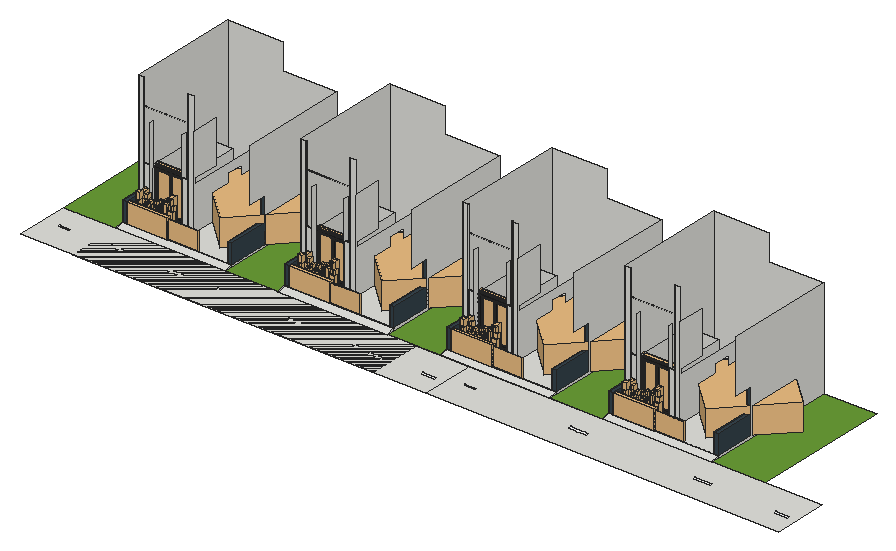
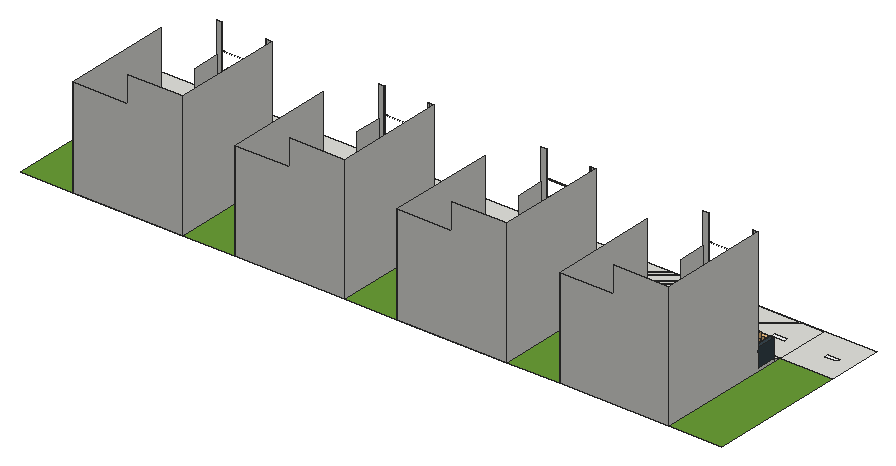
# SketchUp Ruby script. Lengths in inches.
U = 1.inch
M = Sketchup.active_model
def pt(a) = Geom::Point3d.new(a.map { |v| v * U })
def face(e, loops, mat)
  f = e.add_face(loops[0].map { |a| pt(a) })
  loops[1..].each { |l| e.add_face(l.map { |a| pt(a) }).erase! }
  f.material = f.back_material = mat if mat
  f
end
# faces: each face lists its corners as indices into pts; further lists are holes
def faces(e, pts, list, mat = nil) = list.each { |f| face(e, (f[0].is_a?(Array) ? f : [f]).map { |l| l.map { |i| pts[i] } }, mat) }
# xy, xz, yz: faces in a plane at the given z, y or x. An outline is a flat list of corners, or four numbers for a rectangle; further outlines are holes
def ring(l) = l.size == 4 ? [[l[0], l[1]], [l[2], l[1]], [l[2], l[3]], [l[0], l[3]]] : l.each_slice(2).to_a
def flat(e, list, mat, &to3) = list.each { |f| face(e, (f[0].is_a?(Array) ? f : [f]).map { |l| ring(l).map { |u, v| to3.(u, v) } }, mat) }
def xy(e, z, list, mat = nil) = flat(e, list, mat) { |x, y| [x, y, z] }
def xz(e, y, list, mat = nil) = flat(e, list, mat) { |x, z| [x, y, z] }
def yz(e, x, list, mat = nil) = flat(e, list, mat) { |y, z| [x, y, z] }
def lines(e, pts, list) = list.each { |a, b| e.add_line(pt(pts[a]), pt(pts[b])) }
# prism: a flat outline (further loops are holes) pulled along v
def prism(e, loops, v, mat = nil)
  f = face(e, loops, mat); d = Geom::Vector3d.new(v.map { |x| x * U })
  f.pushpull(f.normal.samedirection?(d) ? d.length : -d.length)
end
def box(e, o, s, mat = nil) = prism(e, [[o, [o[0] + s[0], o[1], o[2]], [o[0] + s[0], o[1] + s[1], o[2]], [o[0], o[1] + s[1], o[2]]]], [0, 0, s[2]], mat)
def at(x, y, z, deg = 0) = Geom::Transformation.translation(pt([x, y, z])) * Geom::Transformation.rotation(ORIGIN, Z_AXIS, deg.degrees)
def axes(o, x, y, z) = Geom::Transformation.new([*x, 0, *y, 0, *z, 0, *pt(o).to_a, 1])
def part(name) = M.definitions.add(name)
# library, detail: a bought-in or finely detailed component or shape, given as its bounding box
def library(name, o, s) = part(name).tap { |d| box(d.entities, o, s) }
def detail(e, o, s) = box(e.add_group.entities, o, s)
def put(e, d, t, mat = nil) = e.add_instance(d, t).tap { |i| i.material = mat if mat }
def group(e, t, mat = nil) = e.add_group.tap { |g| g.transformation = t; g.material = mat if mat }.entities
root = M.entities
M.materials.add("1480 AP K099 Starless Night-N").color = [54, 68, 77]
M.materials.add("BANANA_BIG_STVOL_1").color = [93, 83, 53]
M.materials.add("Color_000").color = [255, 255, 255]
M.materials.add("Material60").color = [234, 198, 157]
M.materials.add("POT_TEXTURE_1").color = [172, 172, 172]
M.materials.add("POT_TEXTURE_2").color = [160, 154, 144]
M.materials.add("[Color_009]").color = [33, 33, 33]
M.materials.add("[Color_A01]").color = [253, 112, 112]
M.materials["[Color_A01]"].alpha = 0
M.materials.add("[Grass Dark Green]").color = [106, 157, 55]
M.materials.add("soil1").color = [68, 55, 47]
M.materials.add("wood_1").color = [140, 119, 94]
c1 = part("Untitled")
xy(c1.entities,0,[[[158.81,26.5625,306.06,993.3125],[225.28,357.51,237.28,411.51],[239.71,931.55,251.46,972.3],[233.64,703.93,242.14,755.18],[222.04,66.5,231.29,100.5]]])
xy(c1.entities,0,[[222.04,66.5,231.29,100.5],[225.28,357.51,237.28,411.51],[233.64,703.93,242.14,755.18],[239.71,931.55,251.46,972.3]],"Color_000")
c2 = part("Group\#163")
xy(c2.entities,0,[[0,0,144,382]],"[Grass Dark Green]")
c3 = part("Group\#161")
prism(c3.entities,[[[0,22,6],[0,22,0],[0,0,0]]],[300,0,0])
c4 = library("RANGE ROVER",[-63.71,-35.21,42.76],[182.88,182.88,64.08])
c5 = part("Bilal architect uae abu dhabi ")
put(c5.entities,c4,axes([104.22,-10.75,-48.75],[0.98727,0.57,0],[-0.57,0.98727,0],[0,0,1.14]),"Material60")
c6 = part("Group\#33")
prism(c6.entities,[[[22.64,0,0],[0,0,0],[0,43.31,0],[22.64,43.31,0]],[[20.67,41.34,0],[1.97,41.34,0],[1.97,1.97,0],[20.67,1.97,0]]],[0,0,1.38])
c7 = part("Group\#34")
box(c7.entities,[0,0,0],[18.7,39.37,0.39])
c8 = part("2slidwin w fix bottom")
put(c8.entities,c6,axes([1.97,0,22.15],[1,0,0],[0,0,1.25],[0,-1,0]),"[Color_009]")
put(c8.entities,c7,axes([3.9375,-0.2,24.61],[1,0,0],[0,0,1.25],[0,-1,0]),"[Color_A01]")
g1 = group(c8.entities,at(0,-0.2,0),"[Color_009]")
prism(g1,[[[47.24,0,19.69],[0,0,19.69],[0,0,78.74],[47.24,0,78.74]],[[45.28,0,22.15],[45.28,0,76.28],[1.97,0,76.28],[1.97,0,22.15]]],[0,-3.15,0])
put(c8.entities,c6,axes([22.64,-1.38,22.15],[1,0,0],[0,0,1.25],[0,-1,0]),"[Color_009]")
put(c8.entities,c7,axes([24.61,-1.57,24.61],[1,0,0],[0,0,1.25],[0,-1,0]),"[Color_A01]")
c9 = library("door by lz",[5.91,-4.92,0],[35.43,6.61,78.74])
c10 = library("Modern Gate 1",[0,0,0],[118.11,1.97,78.74])
c11 = library("Window_Curtains2",[0,-81.89,0],[92,82.37,8.12])
c12 = library("Group\#7",[0,-1,0],[111.5625,10,53])
c13 = part("Group")
box(c13.entities,[0,0,0],[12,55.4375,53])
c14 = part("Group\#6")
box(c14.entities,[0,0,0],[12,112.0625,53])
c15 = library("Group\#137",[-640.625,-1318.37,287.11],[396.64,314.81,689.96])
c16 = library("Group\#132",[-513.94,-1201.2,195.17],[480.66,557.42,1160.08])
c17 = library("Group\#134",[-208.03,-1336.63,286.21],[381.72,484.79,1145.39])
c18 = library("Group\#140",[-619.83,-1636.3,288.9],[316.15,456.61,1171.28])
c19 = library("Group\#141",[-738.91,-1210.08,301],[426.4,388.88,1000.79])
c20 = library("Group\#143",[-208.33,-1511.76,297.04],[508.2,421.96,1258.76])
c21 = library("Group\#133",[-545.36,-1775.03,287.125],[412.21,432,920.68])
c22 = library("Group\#138",[-750.24,-1478.51,301.56],[423.84,451.05,998.69])
c23 = library("Group\#136",[-245.33,-1174.2,301.22],[356.02,306.31,608.34])
c24 = library("Group\#131",[-487.23,-1483.58,-4.71],[450.86,446.99,418.38])
c25 = library("Group\#145",[-445.7,-1606.55,154.18],[255.44,283.57,849.28])
c26 = library("Group\#146",[-390.1,-1177.12,195.59],[220.93,265.44,790.12])
c27 = library("Group\#148",[-480.32,-1333.42,295.8],[424.49,356.06,1482.77])
c28 = library("Group\#149",[-378.01,-1245.98,305.66],[422.15,474.55,1267.42])
c29 = library("Group\#135",[-163.65,-1622.09,292.29],[406.18,374.8,780.12])
c30 = library("Group\#144",[-384.8,-1640.99,300.61],[422.68,348.03,1297.96])
c31 = library("Group\#130",[-429.18,-1441.17,362.05],[345.84,348.28,45.35])
c32 = library("Group\#147",[-208.0625,-1498.77,286.27],[547.26,435.76,1075.6])
c33 = library("Group\#142",[-172.82,-1329.68,294.68],[502.85,397.72,955.79])
c34 = library("Group\#139",[-426.76,-1753.59,287.48],[479.67,412.35,1049.19])
c35 = part("Potted palm")
put(c35.entities,c15,at(750.24,1775.03,4.71))
put(c35.entities,c16,at(750.24,1775.03,4.71))
put(c35.entities,c17,at(750.24,1775.03,4.71))
put(c35.entities,c18,at(750.24,1775.03,4.71))
put(c35.entities,c19,at(750.24,1775.03,4.71))
put(c35.entities,c20,at(750.24,1775.03,4.71))
put(c35.entities,c21,at(750.24,1775.03,4.71))
put(c35.entities,c22,at(750.24,1775.03,4.71))
put(c35.entities,c23,at(750.24,1775.03,4.71))
put(c35.entities,c24,at(750.24,1775.03,4.71),"POT_TEXTURE_1")
put(c35.entities,c25,at(750.24,1775.03,4.71))
put(c35.entities,c26,at(750.24,1775.03,4.71))
put(c35.entities,c27,at(750.24,1775.03,4.71))
put(c35.entities,c28,at(750.24,1775.03,4.71))
put(c35.entities,c29,at(750.24,1775.03,4.71))
put(c35.entities,c30,at(750.24,1775.03,4.71))
put(c35.entities,c31,at(750.24,1775.03,4.71),"soil1")
put(c35.entities,c32,at(750.24,1775.03,4.71))
put(c35.entities,c33,at(750.24,1775.03,4.71))
put(c35.entities,c34,at(750.24,1775.03,4.71))
c36 = library("Group\#96",[-662.41,217.3,320.04],[397.32,658.3,1732.06])
c37 = library("Group\#98",[-299.2,181.55,262.58],[360.65,735.71,1258.34])
c38 = library("Group\#93",[-1038.76,656.55,345.34],[733.18,460.51,2065.7])
c39 = library("Group\#91",[-445.29,890.31,329.28],[284.3,304.08,2023.29])
c40 = library("Group\#94",[-733.48,439.625,202.64],[456.28,533.12,1536.78])
c41 = library("Group\#97",[-455.56,899.32,410.78],[341.21,610.33,1581.5])
c42 = library("Group\#90",[-516.34,626.77,-4.5625],[517.73,515.95,418.98])
c43 = library("Group\#95",[-249.24,914.85,310.18],[345.55,647.95,1307.93])
c44 = library("Group\#92",[-277.97,488.68,287.26],[362.84,405.94,1768.54])
c45 = library("Group\#89",[-468.76,669.89,380.1875],[424.36,427.47,41.99])
c46 = part("Potted broadleaf plant")
put(c46.entities,c36,at(1038.76,-181.55,4.5625))
put(c46.entities,c37,at(1038.76,-181.55,4.5625))
put(c46.entities,c38,at(1038.76,-181.55,4.5625))
put(c46.entities,c39,at(1038.76,-181.55,4.5625))
put(c46.entities,c40,at(1038.76,-181.55,4.5625))
put(c46.entities,c41,at(1038.76,-181.55,4.5625))
put(c46.entities,c42,at(1038.76,-181.55,4.5625),"POT_TEXTURE_1")
put(c46.entities,c43,at(1038.76,-181.55,4.5625))
put(c46.entities,c44,at(1038.76,-181.55,4.5625))
put(c46.entities,c45,at(1038.76,-181.55,4.5625),"soil1")
c47 = library("Group\#102",[-246.45,-349.05,558.47],[136.91,100.49,66.1])
c48 = library("Group\#105",[-264.68,-415.73,1484.11],[304.64,209.69,227.41])
c49 = library("Group\#112",[-357.04,-394.18,1447.05],[213.62,306.36,356.95])
c50 = library("Group\#100",[-447.02,-464.95,536.35],[343.73,346.24,39.39])
c51 = library("Group\#101",[-394.9,-448.99,911.74],[90.19,96.88,85.93])
c52 = library("Group\#111",[-424,-312.27,817.53],[158.81,108.06,136.45])
c53 = library("Group\#115",[-409.02,-515.05,915.53],[69.62,77.27,65.47])
c54 = library("Group\#119",[-548.25,-262.82,1459.54],[373.26,352.35,568])
c55 = library("Group\#129",[-492.14,-508.4,-4.15],[433.72,431.71,567.03])
c56 = library("Group\#122",[-293.78,-482.77,597.9],[158.75,112.78,159.87])
c57 = library("Group\#106",[-545.09,-386.51,922.3125],[300.25,219.65,227.33])
c58 = library("Group\#127",[-292.81,-667.38,1418.14],[215.17,356.07,188.87])
c59 = library("Group\#108",[-292.14,-288.9,1281.79],[169.55,204.34,203.36])
c60 = library("Group\#113",[-568.91,-444.37,1285.4],[307.6,179.39,277.93])
c61 = library("Group\#110",[-341.93,-403.49,744.8125],[64.83,96.32,132.15])
c62 = library("Group\#99",[-258.04,-282.68,604.05],[115.53,137.01,52.63])
c63 = library("Group\#107",[-304.79,-269.16,622.65],[82.06,111.89,102.57])
c64 = library("Group\#114",[-388.93,-514.39,838.93],[89.79,77.73,82.08])
c65 = library("Group\#116",[-295.03,-516.52,742.34],[68.71,141.75,78.67])
c66 = library("Group\#123",[-422.77,-235.4,843.61],[178.54,197.77,233.54])
c67 = library("Group\#117",[-498.98,-524.4,908.45],[120.83,107.95,112.98])
c68 = library("Group\#120",[-321.08,-139.66,1308.49],[285.55,393.29,221.53])
c69 = library("Group\#118",[-278.4,-571.99,1530.91],[311.57,345.77,423.62])
c70 = library("Group\#121",[-387.74,-136.11,1470.07],[230,321.58,230.27])
c71 = library("Group\#109",[-244.55,-305.59,1009.46],[103.13,76.81,77.34])
c72 = library("Group\#128",[-385.21,-446.52,494.02],[160.93,321.12,1142.36])
c73 = library("Group\#103",[-249.18,-250.59,980.93],[152.21,116.16,134.05])
c74 = library("Group\#104",[-438.92,-265.61,702.3],[171.52,146.16,133.5])
c75 = part("Potted broadleaf tree")
p = [[568.91,667.38,4.15],[569.91,667.38,4.15],[569.91,668.38,4.15]]
lines(c75.entities,p,[[0,1],[1,2],[2,0]])
put(c75.entities,c47,at(568.91,667.38,4.15))
put(c75.entities,c48,at(568.91,667.38,4.15))
put(c75.entities,c49,at(568.91,667.38,4.15))
put(c75.entities,c50,at(568.91,667.38,4.15),"soil1")
put(c75.entities,c51,at(568.91,667.38,4.15))
put(c75.entities,c52,at(568.91,667.38,4.15))
put(c75.entities,c53,at(568.91,667.38,4.15))
put(c75.entities,c54,at(568.91,667.38,4.15))
put(c75.entities,c55,at(568.91,667.38,4.15),"POT_TEXTURE_2")
put(c75.entities,c56,at(568.91,667.38,4.15))
put(c75.entities,c57,at(568.91,667.38,4.15))
put(c75.entities,c58,at(568.91,667.38,4.15))
put(c75.entities,c59,at(568.91,667.38,4.15))
put(c75.entities,c60,at(568.91,667.38,4.15))
put(c75.entities,c61,at(568.91,667.38,4.15))
put(c75.entities,c62,at(568.91,667.38,4.15))
put(c75.entities,c63,at(568.91,667.38,4.15))
put(c75.entities,c64,at(568.91,667.38,4.15))
put(c75.entities,c65,at(568.91,667.38,4.15))
put(c75.entities,c66,at(568.91,667.38,4.15))
put(c75.entities,c67,at(568.91,667.38,4.15))
put(c75.entities,c68,at(568.91,667.38,4.15))
put(c75.entities,c69,at(568.91,667.38,4.15))
put(c75.entities,c70,at(568.91,667.38,4.15))
put(c75.entities,c71,at(568.91,667.38,4.15))
put(c75.entities,c72,at(568.91,667.38,4.15),"wood_1")
put(c75.entities,c73,at(568.91,667.38,4.15))
put(c75.entities,c74,at(568.91,667.38,4.15))
c76 = library("Group\#150",[-480.3,-2300.47,677.45],[398.14,398.43,28.25])
c77 = library("Group\#151",[-336.38,-2175.79,614.41],[133.99,147.1,560.64])
c78 = library("Group\#152",[-311.45,-2362.85,663.67],[597.01,322.07,1007.38])
c79 = library("Group\#153",[-330.26,-2159.14,612.04],[116.66,119.22,673.97])
c80 = library("Group\#154",[-667.53,-2111.4375,1071.74],[420.02,555.28,968.03])
c81 = library("Group\#155",[-328.97,-2115.58,1156.29],[117.86,119.42,695.38])
c82 = library("Group\#156",[-943.22,-2312.1875,967.59],[670.63,402.45,1245.73])
c83 = library("Group\#158",[-343.93,-2076.42,1024.91],[285.05,475.82,708.21])
c84 = library("Group\#157",[-568.09,-2386.9,-3.76],[573.62,569.18,700.28])
c85 = library("Group\#159",[-550.09,-2664.39,1031.96],[371.42,533.86,798])
c86 = library("Group\#160",[-308.37,-2556.11,869.35],[483.58,483.6,1385.8])
c87 = part("Potted broadleaf plant \#1")
put(c87.entities,c76,at(943.22,2664.39,3.76),"soil1")
put(c87.entities,c77,at(943.22,2664.39,3.76),"BANANA_BIG_STVOL_1")
put(c87.entities,c78,at(943.22,2664.39,3.76))
put(c87.entities,c79,at(943.22,2664.39,3.76),"BANANA_BIG_STVOL_1")
put(c87.entities,c80,at(943.22,2664.39,3.76))
put(c87.entities,c81,at(943.22,2664.39,3.76))
put(c87.entities,c82,at(943.22,2664.39,3.76))
put(c87.entities,c83,at(943.22,2664.39,3.76))
put(c87.entities,c84,at(943.22,2664.39,3.76),"POT_TEXTURE_2")
put(c87.entities,c85,at(943.22,2664.39,3.76))
put(c87.entities,c86,at(943.22,2664.39,3.76))
xy(root,0,[[144,169.25,444,529.25],[588,169.25,888,529.25],[1032,169.25,1332,529.25],[1476,169.25,1776,529.25]])
xy(root,6,[[144,169.25,444,169.25,444,281.3125,432,281.3125,432,481.25,294,481.25,294,472.1875,288,472.1875,288,424.1875,294,424.1875,294,224.6875,279.22,224.6875,279.22,225.16,278.75,225.16,278.75,224.6875,263,224.6875,263,398.125,175,398.125,175,224.6875,159.1,224.6875,159.1,225.16,158.625,225.16,158.625,224.6875,144,224.6875],[588,169.25,888,169.25,888,281.3125,876,281.3125,876,481.25,738,481.25,738,472.1875,732,472.1875,732,424.1875,738,424.1875,738,224.6875,723.22,224.6875,723.22,225.16,722.75,225.16,722.75,224.6875,707,224.6875,707,398.125,619,398.125,619,224.6875,603.1,224.6875,603.1,225.16,602.625,225.16,602.625,224.6875,588,224.6875],[1032,169.25,1332,169.25,1332,281.3125,1320,281.3125,1320,481.25,1182,481.25,1182,472.1875,1176,472.1875,1176,424.1875,1182,424.1875,1182,224.6875,1167.22,224.6875,1167.22,225.16,1166.75,225.16,1166.75,224.6875,1151,224.6875,1151,398.125,1063,398.125,1063,224.6875,1047.1,224.6875,1047.1,225.16,1046.625,225.16,1046.625,224.6875,1032,224.6875],[1476,169.25,1776,169.25,1776,281.3125,1764,281.3125,1764,481.25,1626,481.25,1626,472.1875,1620,472.1875,1620,424.1875,1626,424.1875,1626,224.6875,1611.22,224.6875,1611.22,225.16,1610.75,225.16,1610.75,224.6875,1595,224.6875,1595,398.125,1507,398.125,1507,224.6875,1491.1,224.6875,1491.1,225.16,1490.625,225.16,1490.625,224.6875,1476,224.6875]])
xz(root,169.25,[[144,0,444,6],[588,0,888,6],[1032,0,1332,6],[1476,0,1776,6]])
xz(root,224.6875,[[144,6,158.625,342],[159.1,6,175,132.03],[263,6,278.75,132.03],[279.22,6,294,342],[588,6,602.625,342],
  [603.1,6,619,132.03],[707,6,722.75,132.03],[723.22,6,738,342],[1032,6,1046.625,342],[1047.1,6,1063,132.03],
  [1151,6,1166.75,132.03],[1167.22,6,1182,342],[1476,6,1490.625,342],[1491.1,6,1507,132.03],[1595,6,1610.75,132.03],
  [1611.22,6,1626,342]])
xz(root,225.16,[[158.625,6,159.1,6,159.1,132.03,175,132.03,175,132.5,159.1,132.5,159.1,270.89,215.92,270.89,216.53,270.93,217.15,270.96,217.77,270.98,218.38,271,219.61,271,220.83,270.96,222.05,270.9,222.08,270.89,278.75,270.89,278.75,132.5,263,132.5,263,132.03,278.75,132.03,278.75,6,279.22,6,279.22,342,278.75,342,278.75,271.37,159.1,271.37,159.1,342,158.625,342],[602.625,6,603.1,6,603.1,132.03,619,132.03,619,132.5,603.1,132.5,603.1,270.89,659.92,270.89,660.53,270.93,661.15,270.96,661.77,270.98,662.38,271,663.61,271,664.83,270.96,666.05,270.9,666.08,270.89,722.75,270.89,722.75,132.5,707,132.5,707,132.03,722.75,132.03,722.75,6,723.22,6,723.22,342,722.75,342,722.75,271.37,603.1,271.37,603.1,342,602.625,342],[1046.625,6,1047.1,6,1047.1,132.03,1063,132.03,1063,132.5,1047.1,132.5,1047.1,270.89,1103.92,270.89,1104.53,270.93,1105.15,270.96,1105.77,270.98,1106.38,271,1107.61,271,1108.83,270.96,1110.05,270.9,1110.08,270.89,1166.75,270.89,1166.75,132.5,1151,132.5,1151,132.03,1166.75,132.03,1166.75,6,1167.22,6,1167.22,342,1166.75,342,1166.75,271.37,1047.1,271.37,1047.1,342,1046.625,342],[1490.625,6,1491.1,6,1491.1,132.03,1507,132.03,1507,132.5,1491.1,132.5,1491.1,270.89,1547.92,270.89,1548.53,270.93,1549.15,270.96,1549.77,270.98,1550.38,271,1551.61,271,1552.83,270.96,1554.05,270.9,1554.08,270.89,1610.75,270.89,1610.75,132.5,1595,132.5,1595,132.03,1610.75,132.03,1610.75,6,1611.22,6,1611.22,342,1610.75,342,1610.75,271.37,1491.1,271.37,1491.1,342,1490.625,342]])
xz(root,281.3125,[[432,6,444,126],[876,6,888,126],[1320,6,1332,126],[1764,6,1776,126]],"1480 AP K099 Starless Night-N")
xz(root,398.125,[[175,6,263,126],[619,6,707,126],[1063,6,1151,126],[1507,6,1595,126]])
xz(root,424.1875,[[288,6,294,102],[732,6,738,102],[1176,6,1182,102],[1620,6,1626,102]])
xz(root,472.1875,[[288,6,294,102],[732,6,738,102],[1176,6,1182,102],[1620,6,1626,102]])
xz(root,481.25,[[294,6,432,126],[738,6,876,126],[1182,6,1320,126],[1626,6,1764,126]])
xz(root,529.25,[[144,0,144,342,294,342,294,271,444,271,444,0],[588,0,588,342,738,342,738,271,888,271,888,0],[1032,0,1032,342,1182,342,1182,271,1332,271,1332,0],[1476,0,1476,342,1626,342,1626,271,1776,271,1776,0]])
yz(root,144,[[169.25,0,169.25,6,224.6875,6,224.6875,342,529.25,342,529.25,0]])
yz(root,158.625,[[224.6875,6,225.16,342]])
yz(root,159.1,[[224.6875,6,225.16,132.03]])
yz(root,175,[[224.6875,6,236.25,6,236.25,234.87,224.6875,234.87,224.6875,132.5,225.16,132.5,225.16,132.03,224.6875,132.03],[236.25,6,398.125,126]])
yz(root,263,[[224.6875,6,224.6875,132.03,225.16,132.03,225.16,132.5,224.6875,132.5,224.6875,235.48,236.25,235.48,236.25,6],[236.25,6,398.125,126]])
yz(root,278.75,[[224.6875,6,225.16,132.03]])
yz(root,279.22,[[224.6875,6,225.16,342]])
yz(root,288,[[424.1875,6,472.1875,102]])
yz(root,294,[[[224.6875,6,424.1875,6,424.1875,102,472.1875,102,472.1875,6,481.25,6,481.25,126,229.25,126,229.25,139,301.25,139,301.25,256,224.6875,256],[342.875,54,390.875,102]]])
yz(root,432,[[281.3125,6,481.25,126]])
yz(root,444,[[169.25,0,529.25,0,529.25,271,229.25,271,229.25,126,281.3125,126,281.3125,6,169.25,6]])
yz(root,588,[[169.25,0,169.25,6,224.6875,6,224.6875,342,529.25,342,529.25,0]])
yz(root,602.625,[[224.6875,6,225.16,342]])
yz(root,603.1,[[224.6875,6,225.16,132.03]])
yz(root,619,[[224.6875,6,236.25,6,236.25,234.87,224.6875,234.87,224.6875,132.5,225.16,132.5,225.16,132.03,224.6875,132.03],[236.25,6,398.125,126]])
yz(root,707,[[224.6875,6,224.6875,132.03,225.16,132.03,225.16,132.5,224.6875,132.5,224.6875,235.48,236.25,235.48,236.25,6],[236.25,6,398.125,126]])
yz(root,722.75,[[224.6875,6,225.16,132.03]])
yz(root,723.22,[[224.6875,6,225.16,342]])
yz(root,732,[[424.1875,6,472.1875,102]])
yz(root,738,[[[224.6875,6,424.1875,6,424.1875,102,472.1875,102,472.1875,6,481.25,6,481.25,126,229.25,126,229.25,139,301.25,139,301.25,256,224.6875,256],[342.875,54,390.875,102]]])
yz(root,876,[[281.3125,6,481.25,126]])
yz(root,888,[[169.25,0,529.25,0,529.25,271,229.25,271,229.25,126,281.3125,126,281.3125,6,169.25,6]])
yz(root,1032,[[169.25,0,169.25,6,224.6875,6,224.6875,342,529.25,342,529.25,0]])
yz(root,1046.625,[[224.6875,6,225.16,342]])
yz(root,1047.1,[[224.6875,6,225.16,132.03]])
yz(root,1063,[[224.6875,6,236.25,6,236.25,234.87,224.6875,234.87,224.6875,132.5,225.16,132.5,225.16,132.03,224.6875,132.03],[236.25,6,398.125,126]])
yz(root,1151,[[224.6875,6,224.6875,132.03,225.16,132.03,225.16,132.5,224.6875,132.5,224.6875,235.48,236.25,235.48,236.25,6],[236.25,6,398.125,126]])
yz(root,1166.75,[[224.6875,6,225.16,132.03]])
yz(root,1167.22,[[224.6875,6,225.16,342]])
yz(root,1176,[[424.1875,6,472.1875,102]])
yz(root,1182,[[[224.6875,6,424.1875,6,424.1875,102,472.1875,102,472.1875,6,481.25,6,481.25,126,229.25,126,229.25,139,301.25,139,301.25,256,224.6875,256],[342.875,54,390.875,102]]])
yz(root,1320,[[281.3125,6,481.25,126]])
yz(root,1332,[[169.25,0,529.25,0,529.25,271,229.25,271,229.25,126,281.3125,126,281.3125,6,169.25,6]])
yz(root,1476,[[169.25,0,169.25,6,224.6875,6,224.6875,342,529.25,342,529.25,0]])
yz(root,1490.625,[[224.6875,6,225.16,342]])
yz(root,1491.1,[[224.6875,6,225.16,132.03]])
yz(root,1507,[[224.6875,6,236.25,6,236.25,234.87,224.6875,234.87,224.6875,132.5,225.16,132.5,225.16,132.03,224.6875,132.03],[236.25,6,398.125,126]])
yz(root,1595,[[224.6875,6,224.6875,132.03,225.16,132.03,225.16,132.5,224.6875,132.5,224.6875,235.48,236.25,235.48,236.25,6],[236.25,6,398.125,126]])
yz(root,1610.75,[[224.6875,6,225.16,132.03]])
yz(root,1611.22,[[224.6875,6,225.16,342]])
yz(root,1620,[[424.1875,6,472.1875,102]])
yz(root,1626,[[[224.6875,6,424.1875,6,424.1875,102,472.1875,102,472.1875,6,481.25,6,481.25,126,229.25,126,229.25,139,301.25,139,301.25,256,224.6875,256],[342.875,54,390.875,102]]])
yz(root,1764,[[281.3125,6,481.25,126]])
yz(root,1776,[[169.25,0,529.25,0,529.25,271,229.25,271,229.25,126,281.3125,126,281.3125,6,169.25,6]])
put(root,c1,at(117.4375,306.06,0,-90))
put(root,c1,at(-26.5625,306.06,0,-90))
put(root,c2,at(444,147.25,0))
put(root,c2,at(0,147.25,0))
put(root,c3,at(144,147.25,0))
put(root,c3,at(588,147.25,0))
put(root,c2,at(888,147.25,0))
put(root,c2,at(1332,147.25,0))
put(root,c3,at(1032,147.25,0))
put(root,c3,at(1476,147.25,0))
put(root,c1,at(1084.1875,306.06,0,-90))
put(root,c2,at(1776,147.25,0))
put(root,c5,axes([453.43,441.73,5.875],[-0.2287,-0.9735,0],[-0.9735,0.2287,0],[0,0,1]))
put(root,c5,axes([897.43,441.73,5.875],[-0.2287,-0.9735,0],[-0.9735,0.2287,0],[0,0,1]))
put(root,c5,axes([1341.43,441.73,5.875],[-0.2287,-0.9735,0],[-0.9735,0.2287,0],[0,0,1]))
put(root,c5,axes([1785.43,441.73,5.875],[-0.2287,-0.9735,0],[-0.9735,0.2287,0],[0,0,1]))
put(root,c8,axes([175,243.6,-34],[1.86267,0,0],[0,1.5,0],[0,0,2.032]))
put(root,c8,axes([619,243.6,-34],[1.86267,0,0],[0,1.5,0],[0,0,2.032]))
put(root,c9,axes([288.21,416.14,6],[0,1.36147,0],[-1.21,0,0],[0,0,1.2221]))
put(root,c9,axes([732.21,416.14,6],[0,1.36147,0],[-1.21,0,0],[0,0,1.2221]))
put(root,c10,axes([267.5625,170.86,6],[0.69,0,0],[0,1,0],[0,0,0.62598]))
put(root,c10,axes([711.5625,170.86,6],[0.69,0,0],[0,1,0],[0,0,0.62598]))
put(root,c11,axes([171.28,256.24,125.3],[1.07666,0,0],[0,0,1.45695],[0,-1,0]))
put(root,c12,at(156,169.25,6))
put(root,c13,at(144,169.25,6),"1480 AP K099 Starless Night-N")
put(root,c14,at(432,169.25,6),"1480 AP K099 Starless Night-N")
put(root,c11,axes([615.28,256.24,125.3],[1.07666,0,0],[0,0,1.45695],[0,-1,0]))
put(root,c12,at(600,169.25,6))
put(root,c13,at(588,169.25,6),"1480 AP K099 Starless Night-N")
put(root,c14,at(876,169.25,6),"1480 AP K099 Starless Night-N")
put(root,c35,axes([180.42,214.77,6],[0,-0.0242,0],[0.0242,0,0],[0,0,0.03194]))
put(root,c35,axes([624.42,214.77,6],[0,-0.0242,0],[0.0242,0,0],[0,0,0.03194]))
put(root,c8,axes([1063,243.6,-34],[1.86267,0,0],[0,1.5,0],[0,0,2.032]))
put(root,c8,axes([1507,243.6,-34],[1.86267,0,0],[0,1.5,0],[0,0,2.032]))
put(root,c9,axes([1176.21,416.14,6],[0,1.36147,0],[-1.21,0,0],[0,0,1.2221]))
put(root,c9,axes([1620.21,416.14,6],[0,1.36147,0],[-1.21,0,0],[0,0,1.2221]))
put(root,c10,axes([1155.5625,170.86,6],[0.69,0,0],[0,1,0],[0,0,0.62598]))
put(root,c10,axes([1599.5625,170.86,6],[0.69,0,0],[0,1,0],[0,0,0.62598]))
put(root,c11,axes([1059.28,256.24,125.3],[1.07666,0,0],[0,0,1.45695],[0,-1,0]))
put(root,c12,at(1044,169.25,6))
put(root,c13,at(1032,169.25,6),"1480 AP K099 Starless Night-N")
put(root,c14,at(1320,169.25,6),"1480 AP K099 Starless Night-N")
put(root,c11,axes([1503.28,256.24,125.3],[1.07666,0,0],[0,0,1.45695],[0,-1,0]))
put(root,c12,at(1488,169.25,6))
put(root,c13,at(1476,169.25,6),"1480 AP K099 Starless Night-N")
put(root,c14,at(1764,169.25,6),"1480 AP K099 Starless Night-N")
put(root,c35,axes([1068.42,214.77,6],[0,-0.0242,0],[0.0242,0,0],[0,0,0.03194]))
put(root,c35,axes([1512.42,214.77,6],[0,-0.0242,0],[0.0242,0,0],[0,0,0.03194]))
put(root,c46,axes([227.77,221.75,6],[0,-0.0242,0],[0.0242,0,0],[0,0,0.03194]))
put(root,c46,axes([671.77,221.75,6],[0,-0.0242,0],[0.0242,0,0],[0,0,0.03194]))
put(root,c46,axes([1115.77,221.75,6],[0,-0.0242,0],[0.0242,0,0],[0,0,0.03194]))
put(root,c46,axes([1559.77,221.75,6],[0,-0.0242,0],[0.0242,0,0],[0,0,0.03194]))
put(root,c75,axes([207.22,210.38,6.02],[0,-0.0242,0],[0.0242,0,0],[0,0,0.03194]))
put(root,c75,axes([651.22,210.38,6.02],[0,-0.0242,0],[0.0242,0,0],[0,0,0.03194]))
put(root,c75,axes([1095.22,210.38,6.02],[0,-0.0242,0],[0.0242,0,0],[0,0,0.03194]))
put(root,c75,axes([1539.22,210.38,6.02],[0,-0.0242,0],[0.0242,0,0],[0,0,0.03194]))
put(root,c87,axes([158.9,219.44,6.03],[0,-0.0242,0],[0.0242,0,0],[0,0,0.03194]))
put(root,c87,axes([602.9,219.44,6.03],[0,-0.0242,0],[0.0242,0,0],[0,0,0.03194]))
put(root,c87,axes([1046.9,219.44,6.03],[0,-0.0242,0],[0.0242,0,0],[0,0,0.03194]))
put(root,c87,axes([1490.9,219.44,6.03],[0,-0.0242,0],[0.0242,0,0],[0,0,0.03194]))
